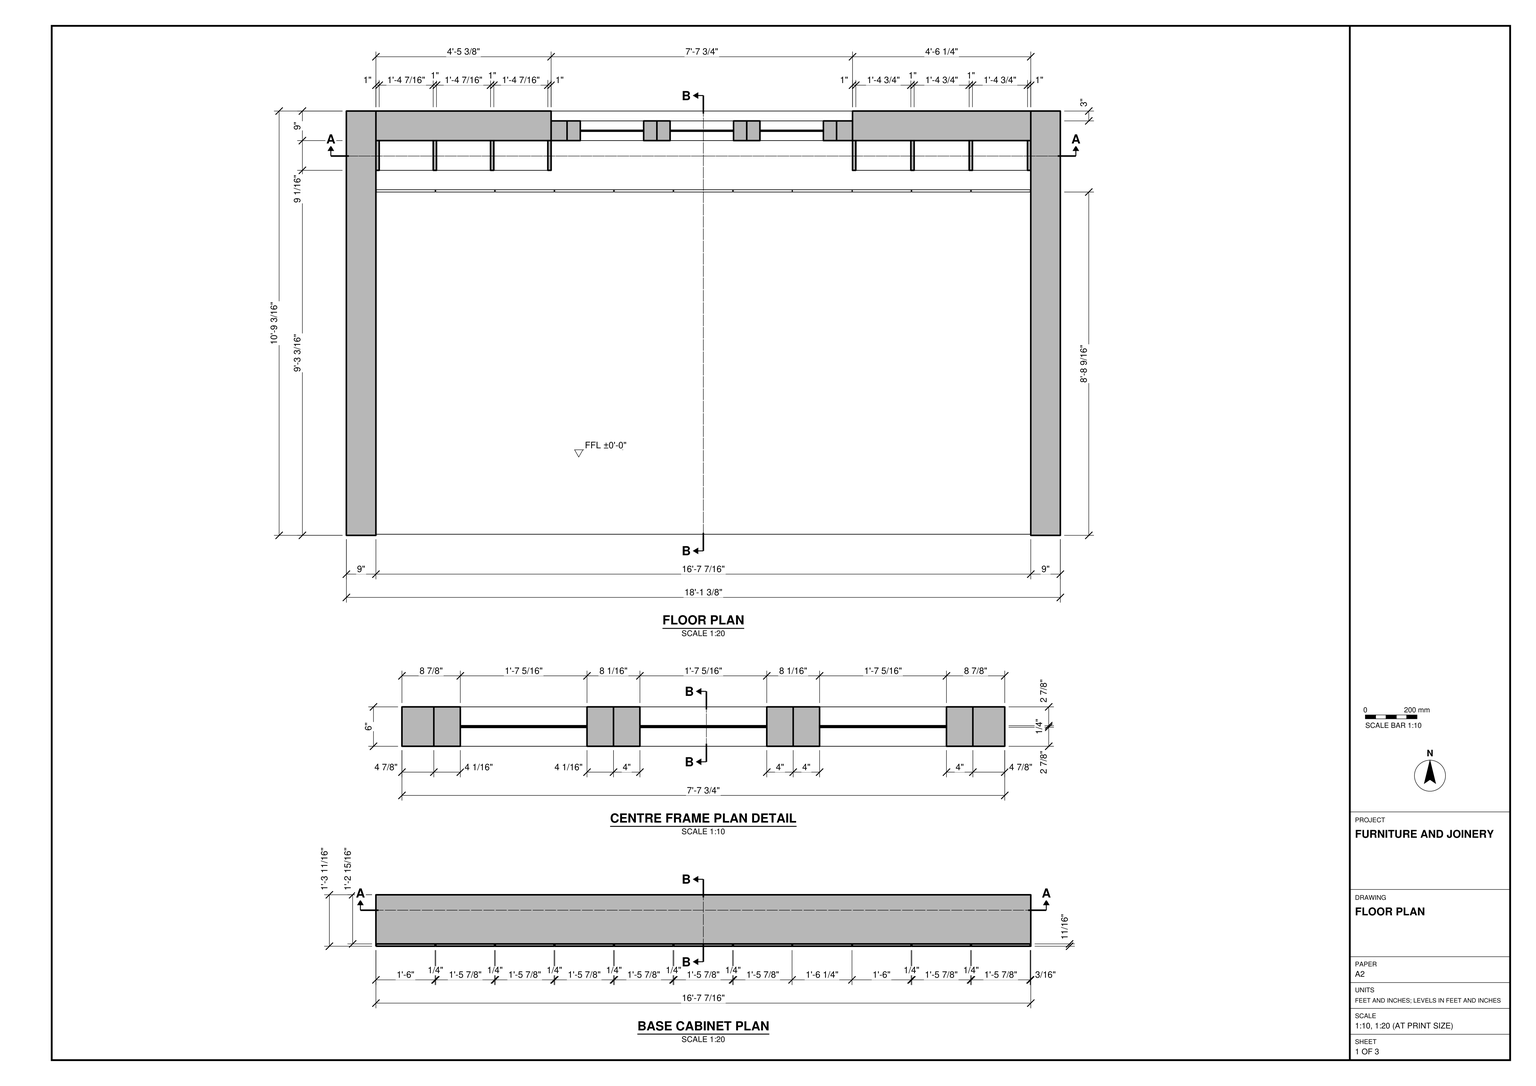
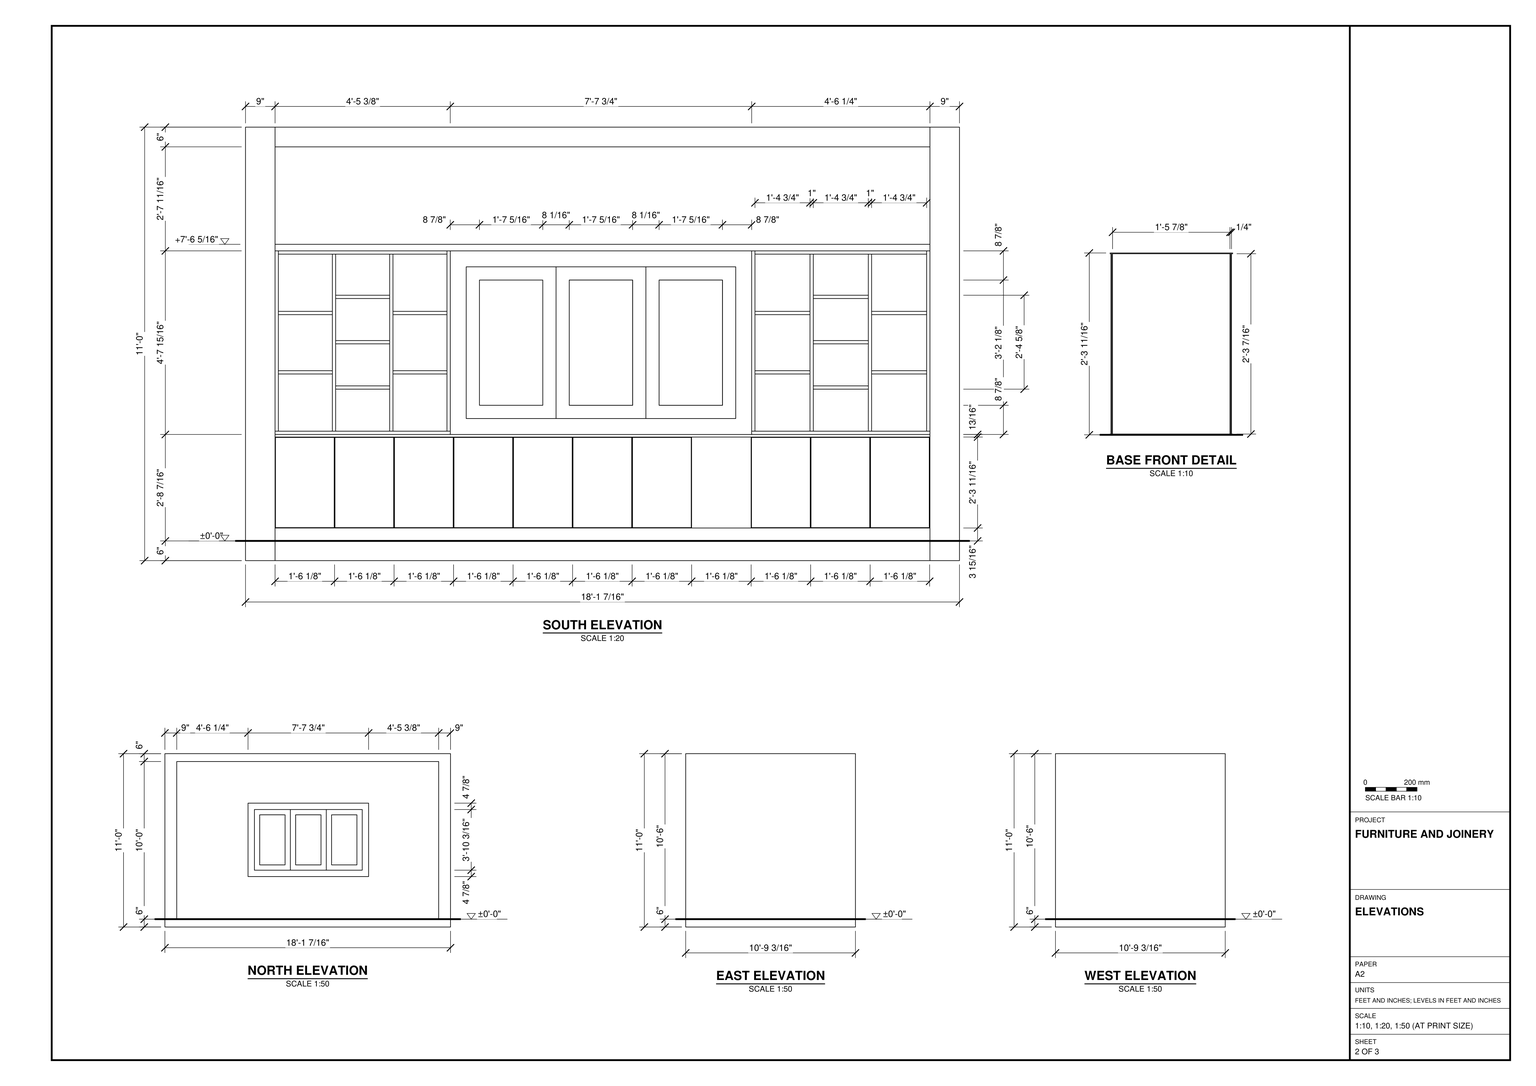
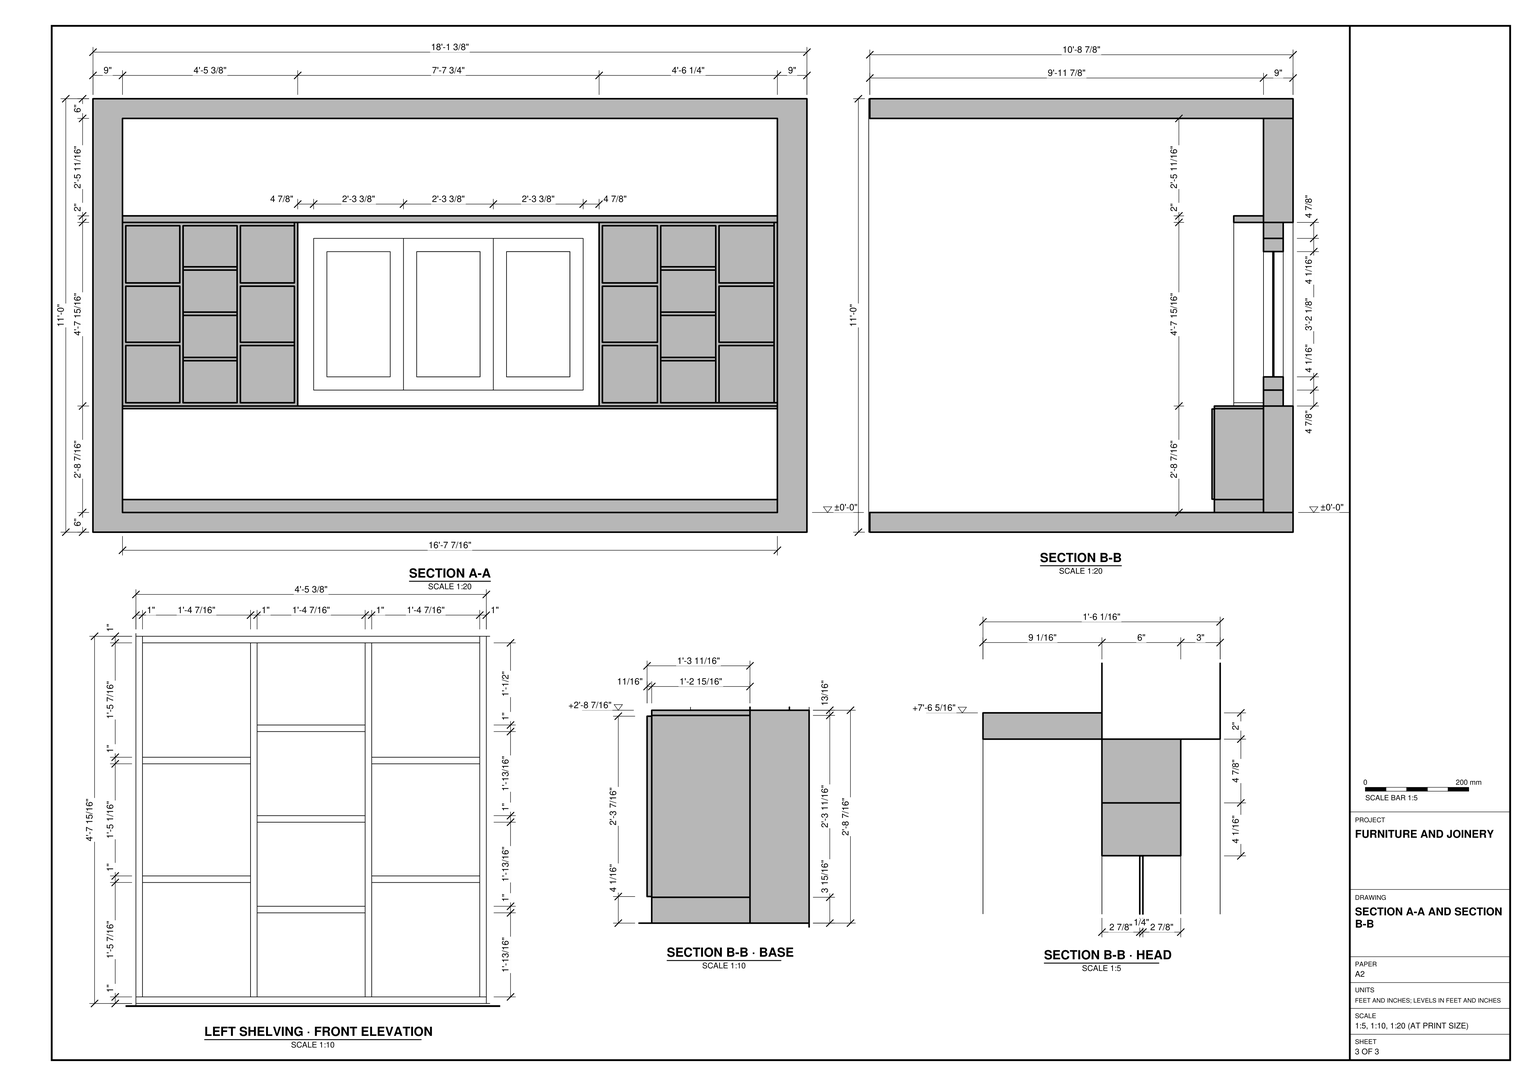
Use task_files/diagram_01.pdf to model the built-in joinery and its surrounding shell in SketchUp. Work in feet and inches. The overall model is 18'-1 7/16" wide, 10'-9 3/16" deep and 11'-0" high. Set the finished floor at ±0'-0". Model the floor slab, the two side walls, the back wall with its window opening, and the roof slab. Leave the front open as drawn.

Run the base cabinet between the side walls. Use the base plan and section to set the depth of its top, the projection of its fronts and the setback of its plinth. Above the base, fit open shelving on either side of the central window. Follow the separate widths shown for the left and right shelving units rather than making them identical. In each unit, align the shelves in the outer bays and use the closer shelf spacing shown in the middle bay. Use the centre frame plan and head section to place the glazing within the frame and set the projection of the continuous head board.

Keep the shell elements and each joinery piece in separate groups or components, and use components for repeated parts. Any decor or loose items may be suitable library components. Save one SketchUp model as output_files/built_in_cabinet_wall_around_a_three_panel_window.skp.

# SketchUp Ruby script. Lengths in inches.
U = 1.inch
M = Sketchup.active_model
def pt(a) = Geom::Point3d.new(a.map { |v| v * U })
def face(e, loops, mat)
  f = e.add_face(loops[0].map { |a| pt(a) })
  loops[1..].each { |l| e.add_face(l.map { |a| pt(a) }).erase! }
  f.material = f.back_material = mat if mat
  f
end
# faces: each face lists its corners as indices into pts; further lists are holes
def faces(e, pts, list, mat = nil) = list.each { |f| face(e, (f[0].is_a?(Array) ? f : [f]).map { |l| l.map { |i| pts[i] } }, mat) }
# xy, xz, yz: faces in a plane at the given z, y or x. An outline is a flat list of corners, or four numbers for a rectangle; further outlines are holes
def ring(l) = l.size == 4 ? [[l[0], l[1]], [l[2], l[1]], [l[2], l[3]], [l[0], l[3]]] : l.each_slice(2).to_a
def flat(e, list, mat, &to3) = list.each { |f| face(e, (f[0].is_a?(Array) ? f : [f]).map { |l| ring(l).map { |u, v| to3.(u, v) } }, mat) }
def xy(e, z, list, mat = nil) = flat(e, list, mat) { |x, y| [x, y, z] }
def xz(e, y, list, mat = nil) = flat(e, list, mat) { |x, z| [x, y, z] }
def yz(e, x, list, mat = nil) = flat(e, list, mat) { |y, z| [x, y, z] }
def lines(e, pts, list) = list.each { |a, b| e.add_line(pt(pts[a]), pt(pts[b])) }
# prism: a flat outline (further loops are holes) pulled along v
def prism(e, loops, v, mat = nil)
  f = face(e, loops, mat); d = Geom::Vector3d.new(v.map { |x| x * U })
  f.pushpull(f.normal.samedirection?(d) ? d.length : -d.length)
end
def box(e, o, s, mat = nil) = prism(e, [[o, [o[0] + s[0], o[1], o[2]], [o[0] + s[0], o[1] + s[1], o[2]], [o[0], o[1] + s[1], o[2]]]], [0, 0, s[2]], mat)
def at(x, y, z, deg = 0) = Geom::Transformation.translation(pt([x, y, z])) * Geom::Transformation.rotation(ORIGIN, Z_AXIS, deg.degrees)
def axes(o, x, y, z) = Geom::Transformation.new([*x, 0, *y, 0, *z, 0, *pt(o).to_a, 1])
def part(name) = M.definitions.add(name)
# library, detail: a bought-in or finely detailed component or shape, given as its bounding box
def library(name, o, s) = part(name).tap { |d| box(d.entities, o, s) }
def detail(e, o, s) = box(e.add_group.entities, o, s)
def put(e, d, t, mat = nil) = e.add_instance(d, t).tap { |i| i.material = mat if mat }
def group(e, t, mat = nil) = e.add_group.tap { |g| g.transformation = t; g.material = mat if mat }.entities
root = M.entities
M.materials.add("[Color A01]").color = [255, 204, 204]
M.materials.add("[Color B01]").color = [255, 216, 204]
M.materials.add("[Color H07]").color = [0, 153, 153]
M.materials.add("[Polished Concrete New]").color = [200, 200, 203]
M.materials.add("[Translucent Glass Blue]").color = [100, 149, 237]
M.materials["[Translucent Glass Blue]"].alpha = 0.5
M.materials.add("[Wax 01]").color = [250, 213, 163]
M.materials.add("[Wood Board Cork]").color = [215, 201, 115]
c1 = part("Group\#17")
box(c1.entities,[0,0,0],[19.29,0.24,38.13])
c2 = part("Union")
xy(c2.entities,0,[[0,0,0,129.21,217.41,129.21,217.41,0,208.41,0,208.41,0.34,9,0.34,9,0]])
xy(c2.entities,6,[[9,0.34,208.41,129.21]],"[Wax 01]")
xy(c2.entities,126,[[9,0.34,208.41,129.21]],"[Color B01]")
xy(c2.entities,132,[[0,0,9,0,9,0.34,208.41,0.34,208.41,0,217.41,0,217.41,129.21,0,129.21]],"[Polished Concrete New]")
xz(c2.entities,0,[[0,0,9,132],[208.41,0,217.41,132]])
xz(c2.entities,0.34,[[9,0,208.41,6],[9,126,208.41,132]])
xz(c2.entities,129.21,[[[0,0,217.41,132],[9,6,208.41,126]]])
yz(c2.entities,0,[[0,0,129.21,132]])
yz(c2.entities,9,[[0,0,0.34,0,0.34,6,129.21,6,129.21,126,0.34,126,0.34,132,0,132]],"[Color B01]")
yz(c2.entities,208.41,[[0,0,0,132,0.34,132,0.34,126,129.21,126,129.21,6,0.34,6,0.34,0]],"[Color A01]")
yz(c2.entities,217.41,[[0,0,129.21,132]])
xy(root,120.8,[[9,111.16,208.41,120.21]],"[Wood Board Cork]")
xy(root,122.8,[[9,111.16,208.41,120.21]],"[Wood Board Cork]")
xz(root,111.16,[[9,120.8,208.41,122.8]],"[Wood Board Cork]")
xz(root,120.21,[[9,120.8,208.41,122.8]])
yz(root,9,[[111.16,120.8,120.21,122.8]])
yz(root,208.41,[[111.16,120.8,120.21,122.8]])
p = [[62.35,120.21,120.8],[62.35,129.21,120.8],[62.35,120.21,64.89],[62.35,129.21,64.89],[154.13,120.21,120.8],[154.13,129.21,120.8],
  [154.13,120.21,64.89],[154.13,129.21,64.89]]
lines(root,p,[[0,1],[2,3],[4,5],[6,7],[2,0],[6,2],[4,6]])
g1 = group(root,at(9,120.21,32.47),"[Color H07]")
xy(g1,0,[[0,0,199.41,9]])
xy(g1,32.41,[[53.35,0,145.13,9]])
xy(g1,88.32,[[53.35,0,145.13,9]])
xy(g1,120,[[0,0,199.41,9]])
xz(g1,0,[[[0,0,199.41,120],[53.35,32.41,145.13,88.32]]],"[Color H07]")
xz(g1,9,[[[0,0,199.41,120],[53.35,32.41,145.13,88.32]]])
yz(g1,0,[[0,0,9,120]])
yz(g1,53.35,[[0,32.41,9,88.32]])
yz(g1,145.13,[[0,32.41,9,88.32]])
yz(g1,199.41,[[0,0,9,120]])
g2 = group(root,at(9,105.25,32.47),"[Wood Board Cork]")
xy(g2,0,[[0,0,199.41,14.96]])
xy(g2,3.9375,[[0,0,199.41,14.96]])
xy(g2,31.63,[[0,0,199.41,14.96]])
xy(g2,32.41,[[0,0,199.41,14.96]])
xz(g2,0,[[0,0,199.41,3.9375],[0,3.9375,199.41,31.63],[0,31.63,199.41,32.41]])
xz(g2,14.96,[[0,0,199.41,3.9375],[0,3.9375,199.41,31.63],[0,31.63,199.41,32.41]])
yz(g2,0,[[0,0,14.96,3.9375],[0,3.9375,14.96,31.63],[0,31.63,14.96,32.41]])
yz(g2,199.41,[[0,0,14.96,3.9375],[0,3.9375,14.96,31.63],[0,31.63,14.96,32.41]])
g3 = group(root,at(9,120.21,64.89),"[Wood Board Cork]")
xy(g3,0,[[0,-9.06,53.35,0]])
xy(g3,1,[[1,-9.06,17.45,0],[18.45,-9.06,34.9,0],[35.9,-9.06,52.35,0]])
xy(g3,18.42,[[1,-9.06,17.45,0],[35.9,-9.06,52.35,0]])
xy(g3,19.42,[[1,-9.06,17.45,0],[35.9,-9.06,52.35,0]])
xy(g3,36.49,[[1,-9.06,17.45,0],[35.9,-9.06,52.35,0]])
xy(g3,37.49,[[1,-9.06,17.45,0],[35.9,-9.06,52.35,0]])
xy(g3,54.91,[[1,-9.06,17.45,0],[18.45,-9.06,34.9,0],[35.9,-9.06,52.35,0]])
xy(g3,55.91,[[0,-9.06,1,0],[1,-9.06,52.35,0],[52.35,-9.06,53.35,0]])
xz(g3,-9.06,[[0,0,53.35,1],[0,1,1,55.91],[17.45,1,18.45,54.91],[34.9,1,35.9,54.91],[52.35,1,53.35,55.91],
  [1,18.42,17.45,19.42],[35.9,18.42,52.35,19.42],[1,36.49,17.45,37.49],[35.9,36.49,52.35,37.49],[1,54.91,52.35,55.91]])
xz(g3,0,[[52.35,1,53.35,55.91]])
yz(g3,0,[[-9.06,0,0,1],[-9.06,1,0,55.91]])
yz(g3,1,[[-9.06,1,0,18.42],[-9.06,19.42,0,36.49],[-9.06,37.49,0,54.91]])
yz(g3,17.45,[[-9.06,1,0,18.42],[-9.06,19.42,0,36.49],[-9.06,37.49,0,54.91]])
yz(g3,18.45,[[-9.06,1,0,54.91]])
yz(g3,34.9,[[-9.06,1,0,54.91]])
yz(g3,35.9,[[-9.06,1,0,18.42],[-9.06,19.42,0,36.49],[-9.06,37.49,0,54.91]])
yz(g3,52.35,[[-9.06,1,0,18.42],[-9.06,18.42,0,19.42],[-9.06,19.42,0,36.49],[-9.06,37.49,0,54.91],[-9.06,54.91,0,55.91]])
yz(g3,53.35,[[-9.06,0,0,1],[-9.06,1,0,55.91]])
g4 = group(root,at(154.13,120.21,64.89),"[Wood Board Cork]")
xy(g4,0,[[0,-9.06,54.28,0]])
xy(g4,1,[[1,-9.06,17.76,0],[18.76,-9.06,35.52,0],[35.52,-9.06,36.52,0],[36.52,-9.06,53.28,0],[53.28,-9.06,54.28,0]])
xy(g4,18.42,[[1,-9.06,17.76,0],[36.52,-9.06,53.28,0]])
xy(g4,19.42,[[1,-9.06,17.76,0],[36.52,-9.06,53.28,0]])
xy(g4,36.49,[[1,-9.06,17.76,0],[36.52,-9.06,53.28,0]])
xy(g4,37.49,[[1,-9.06,17.76,0],[36.52,-9.06,53.28,0]])
xy(g4,54.91,[[1,-9.06,17.76,0],[18.76,-9.06,35.52,0],[36.52,-9.06,53.28,0]])
xy(g4,55.91,[[0,-9.06,1,0],[1,-9.06,53.28,0],[53.28,-9.06,54.28,0]])
xz(g4,-9.06,[[0,0,54.28,1],[0,1,1,55.91],[17.76,1,18.76,54.91],[35.52,1,36.52,54.91],[53.28,1,54.28,55.91],
  [1,18.42,17.76,19.42],[36.52,18.42,53.28,19.42],[1,36.49,17.76,37.49],[36.52,36.49,53.28,37.49],[1,54.91,53.28,55.91]])
xz(g4,0,[[0,0,54.28,1],[53.28,1,54.28,55.91]])
yz(g4,0,[[-9.06,0,0,1],[-9.06,1,0,55.91]])
yz(g4,1,[[-9.06,1,0,18.42],[-9.06,19.42,0,36.49],[-9.06,37.49,0,54.91]])
yz(g4,17.76,[[-9.06,1,0,18.42],[-9.06,19.42,0,36.49],[-9.06,37.49,0,54.91]])
yz(g4,18.76,[[-9.06,1,0,54.91]])
yz(g4,35.52,[[-9.06,1,0,54.91]])
yz(g4,36.52,[[-9.06,1,0,18.42],[-9.06,19.42,0,36.49],[-9.06,37.49,0,54.91]])
yz(g4,53.28,[[-9.06,1,0,18.42],[-9.06,18.42,0,19.42],[-9.06,19.42,0,36.49],[-9.06,36.49,0,37.49],[-9.06,37.49,0,54.91],
  [-9.06,54.91,0,55.91]])
yz(g4,54.28,[[-9.06,0,0,1],[-9.06,1,0,55.91]])
g5 = group(root,at(27.45,120.21,106.29),"[Wood Board Cork]")
box(g5,[0,-9.06,0],[16.45,9.06,1])
box(g5,[0,-9.06,-13.8],[16.45,9.06,1])
box(g5,[0,-9.06,-27.6],[16.45,9.06,1])
box(g5,[145.44,-9.06,0],[16.76,9.06,1])
box(g5,[145.44,-9.06,-13.8],[16.76,9.06,1])
box(g5,[145.44,-9.06,-27.6],[16.76,9.06,1])
g6 = group(root,at(9,105.25,36.41))
xy(g6,0.12,[[0.12,-0.71,18,0]])
xy(g6,27.57,[[0.12,-0.71,18,0]])
xz(g6,-0.71,[[0.12,0.12,18,27.57]])
xz(g6,0,[[[0,0,18.12,27.69],[0.12,0.12,18,27.57]]])
yz(g6,0.12,[[-0.71,0.12,0,27.57]])
yz(g6,18,[[-0.71,0.12,0,27.57]])
g7 = group(root,at(27.12,105.25,36.41))
xy(g7,0.12,[[0.12,-0.71,18,0]])
xy(g7,27.57,[[0.12,-0.71,18,0]])
xz(g7,-0.71,[[0.12,0.12,18,27.57]])
xz(g7,0,[[[0,0,18.12,27.69],[0.12,0.12,18,27.57]]])
yz(g7,0.12,[[-0.71,0.12,0,27.57]])
yz(g7,18,[[-0.71,0.12,0,27.57]])
g8 = group(root,at(45.24,105.25,36.41))
xy(g8,0.12,[[0.12,-0.71,18,0]])
xy(g8,27.57,[[0.12,-0.71,18,0]])
xz(g8,-0.71,[[0.12,0.12,18,27.57]])
xz(g8,0,[[[0,0,18.12,27.69],[0.12,0.12,18,27.57]]])
yz(g8,0.12,[[-0.71,0.12,0,27.57]])
yz(g8,18,[[-0.71,0.12,0,27.57]])
g9 = group(root,at(63.36,105.25,36.41))
xy(g9,0.12,[[0.12,-0.71,18,0]])
xy(g9,27.57,[[0.12,-0.71,18,0]])
xz(g9,-0.71,[[0.12,0.12,18,27.57]])
xz(g9,0,[[[0,0,18.12,27.69],[0.12,0.12,18,27.57]]])
yz(g9,0.12,[[-0.71,0.12,0,27.57]])
yz(g9,18,[[-0.71,0.12,0,27.57]])
g10 = group(root,at(81.48,105.25,36.41))
xy(g10,0.12,[[0.12,-0.71,18,0]])
xy(g10,27.57,[[0.12,-0.71,18,0]])
xz(g10,-0.71,[[0.12,0.12,18,27.57]])
xz(g10,0,[[[0,0,18.12,27.69],[0.12,0.12,18,27.57]]])
yz(g10,0.12,[[-0.71,0.12,0,27.57]])
yz(g10,18,[[-0.71,0.12,0,27.57]])
g11 = group(root,at(99.6,105.25,36.41))
xy(g11,0.12,[[0.12,-0.71,18,0]])
xy(g11,27.57,[[0.12,-0.71,18,0]])
xz(g11,-0.71,[[0.12,0.12,18,27.57]])
xz(g11,0,[[[0,0,18.12,27.69],[0.12,0.12,18,27.57]]])
yz(g11,0.12,[[-0.71,0.12,0,27.57]])
yz(g11,18,[[-0.71,0.12,0,27.57]])
g12 = group(root,at(117.72,105.25,36.41))
xy(g12,0.12,[[0.12,-0.71,18,0]])
xy(g12,27.57,[[0.12,-0.71,18,0]])
xz(g12,-0.71,[[0.12,0.12,18,27.57]])
xz(g12,0,[[[0,0,18.12,27.69],[0.12,0.12,18,27.57]]])
yz(g12,0.12,[[-0.71,0.12,0,27.57]])
yz(g12,18,[[-0.71,0.12,0,27.57]])
g13 = group(root,at(135.84,105.25,36.41))
box(g13,[0,-0.71,0],[18.12,0.71,27.69])
g14 = group(root,at(153.96,105.25,36.41))
xy(g14,0.12,[[0.12,-0.71,18,0]])
xy(g14,27.57,[[0.12,-0.71,18,0]])
xz(g14,-0.71,[[0.12,0.12,18,27.57]])
xz(g14,0,[[[0,0,18.12,27.69],[0.12,0.12,18,27.57]]])
yz(g14,0.12,[[-0.71,0.12,0,27.57]])
yz(g14,18,[[-0.71,0.12,0,27.57]])
g15 = group(root,at(172.08,105.25,36.41))
xy(g15,0.12,[[0.12,-0.71,18,0]])
xy(g15,27.57,[[0.12,-0.71,18,0]])
xz(g15,-0.71,[[0.12,0.12,18,27.57]])
xz(g15,0,[[[0,0,18.12,27.69],[0.12,0.12,18,27.57]]])
yz(g15,0.12,[[-0.71,0.12,0,27.57]])
yz(g15,18,[[-0.71,0.12,0,27.57]])
g16 = group(root,at(190.2,105.25,36.41))
xy(g16,0.12,[[0.12,-0.71,18,0]])
xy(g16,27.57,[[0.12,-0.71,18,0]])
xz(g16,-0.71,[[0.12,0.12,18,27.57]])
xz(g16,0,[[[0,0,18.12,27.69],[0.12,0.12,18,27.57]]])
yz(g16,0.12,[[-0.71,0.12,0,27.57]])
yz(g16,18,[[-0.71,0.12,0,27.57]])
g17 = group(root,at(62.35,120.21,64.89))
xy(g17,0,[[0,0,91.78,6]])
xy(g17,4.86,[[4.86,0,32.21,6],[32.21,0,59.57,6],[59.57,0,86.92,6]])
xy(g17,8.875,[[36.23,0,55.55,6],[63.59,0,82.9,6]])
xy(g17,8.89,[[8.89,0,28.18,6]])
xy(g17,47.02,[[8.89,0,28.18,6]])
xy(g17,47.03,[[36.23,0,55.55,6],[63.59,0,82.9,6]])
xy(g17,51.05,[[4.86,0,32.21,6],[32.21,0,59.57,6],[59.57,0,86.92,6]])
xy(g17,55.91,[[0,0,91.78,6]])
xz(g17,0,[[[0,0,91.78,55.91],[4.86,4.86,86.92,51.05]],[[4.86,4.86,32.21,51.05],[8.89,8.89,28.18,47.02]],[[32.21,4.86,59.57,51.05],[36.23,8.875,55.55,47.03]],[[59.57,4.86,86.92,51.05],[63.59,8.875,82.9,47.03]]])
xz(g17,6,[[[0,0,91.78,55.91],[4.86,4.86,86.92,51.05]],[[4.86,4.86,32.21,51.05],[8.89,8.89,28.18,47.02]],[[32.21,4.86,59.57,51.05],[36.23,8.875,55.55,47.03]],[[59.57,4.86,86.92,51.05],[63.59,8.875,82.9,47.03]]])
yz(g17,0,[[0,0,6,55.91]])
yz(g17,4.86,[[0,4.86,6,51.05]])
yz(g17,8.89,[[0,8.89,6,47.02]])
yz(g17,28.18,[[0,8.89,6,47.02]])
yz(g17,32.21,[[0,4.86,6,51.05]])
yz(g17,36.23,[[0,8.875,6,47.03]])
yz(g17,55.55,[[0,8.875,6,47.03]])
yz(g17,59.57,[[0,4.86,6,51.05]])
yz(g17,63.59,[[0,8.875,6,47.03]])
yz(g17,82.9,[[0,8.875,6,47.03]])
yz(g17,86.92,[[0,4.86,6,51.05]])
yz(g17,91.78,[[0,0,6,55.91]])
put(root,c1,at(71.24,123.1,73.78),"[Translucent Glass Blue]")
put(root,c1,at(98.58,123.1,73.78),"[Translucent Glass Blue]")
put(root,c1,at(125.9375,123.1,73.78),"[Translucent Glass Blue]")
put(root,c2,at(0,0,26.47))
